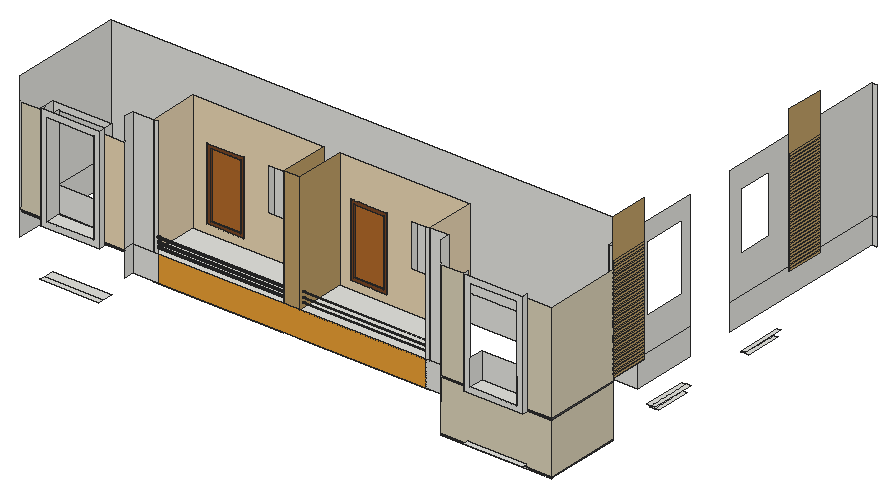
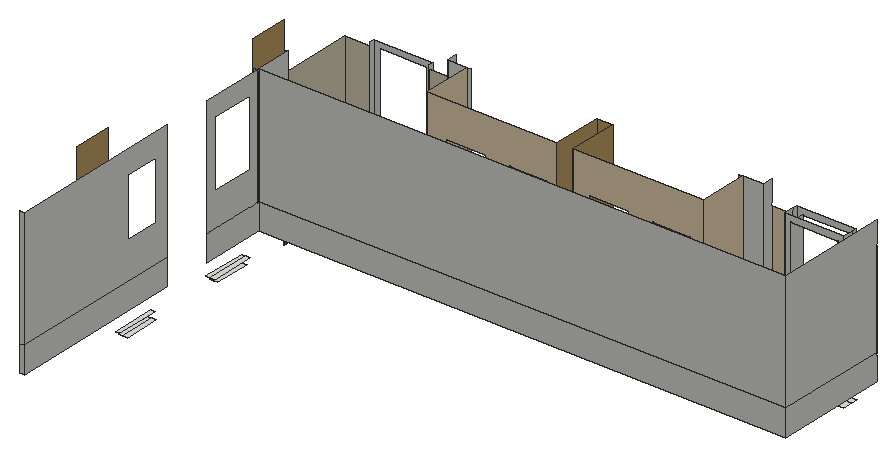
# SketchUp Ruby script. Lengths in inches.
U = 1.inch
M = Sketchup.active_model
def pt(a) = Geom::Point3d.new(a.map { |v| v * U })
def face(e, loops, mat)
  f = e.add_face(loops[0].map { |a| pt(a) })
  loops[1..].each { |l| e.add_face(l.map { |a| pt(a) }).erase! }
  f.material = f.back_material = mat if mat
  f
end
# faces: each face lists its corners as indices into pts; further lists are holes
def faces(e, pts, list, mat = nil) = list.each { |f| face(e, (f[0].is_a?(Array) ? f : [f]).map { |l| l.map { |i| pts[i] } }, mat) }
# xy, xz, yz: faces in a plane at the given z, y or x. An outline is a flat list of corners, or four numbers for a rectangle; further outlines are holes
def ring(l) = l.size == 4 ? [[l[0], l[1]], [l[2], l[1]], [l[2], l[3]], [l[0], l[3]]] : l.each_slice(2).to_a
def flat(e, list, mat, &to3) = list.each { |f| face(e, (f[0].is_a?(Array) ? f : [f]).map { |l| ring(l).map { |u, v| to3.(u, v) } }, mat) }
def xy(e, z, list, mat = nil) = flat(e, list, mat) { |x, y| [x, y, z] }
def xz(e, y, list, mat = nil) = flat(e, list, mat) { |x, z| [x, y, z] }
def yz(e, x, list, mat = nil) = flat(e, list, mat) { |y, z| [x, y, z] }
def lines(e, pts, list) = list.each { |a, b| e.add_line(pt(pts[a]), pt(pts[b])) }
# prism: a flat outline (further loops are holes) pulled along v
def prism(e, loops, v, mat = nil)
  f = face(e, loops, mat); d = Geom::Vector3d.new(v.map { |x| x * U })
  f.pushpull(f.normal.samedirection?(d) ? d.length : -d.length)
end
def box(e, o, s, mat = nil) = prism(e, [[o, [o[0] + s[0], o[1], o[2]], [o[0] + s[0], o[1] + s[1], o[2]], [o[0], o[1] + s[1], o[2]]]], [0, 0, s[2]], mat)
def at(x, y, z, deg = 0) = Geom::Transformation.translation(pt([x, y, z])) * Geom::Transformation.rotation(ORIGIN, Z_AXIS, deg.degrees)
def axes(o, x, y, z) = Geom::Transformation.new([*x, 0, *y, 0, *z, 0, *pt(o).to_a, 1])
def part(name) = M.definitions.add(name)
# library, detail: a bought-in or finely detailed component or shape, given as its bounding box
def library(name, o, s) = part(name).tap { |d| box(d.entities, o, s) }
def detail(e, o, s) = box(e.add_group.entities, o, s)
def put(e, d, t, mat = nil) = e.add_instance(d, t).tap { |i| i.material = mat if mat }
def group(e, t, mat = nil) = e.add_group.tap { |g| g.transformation = t; g.material = mat if mat }.entities
root = M.entities
M.materials.add("Generic").color = [191, 159, 103]
M.materials.add("Generic\#1").color = [233, 159, 52]
M.materials.add("Generic\#2").color = [235, 215, 180]
M.materials.add("Generic\#3").color = [218, 209, 183]
M.materials.add("[Color M06]").color = [86, 86, 86]
M.materials.add("[Wood Bamboo]").color = [177, 105, 43]
M.materials.add("[Wood Veneer 01]").color = [120, 70, 37]
c1 = part("Group\#5")
xy(c1.entities,0,[[0,0,1,57.75]])
xy(c1.entities,2.57,[[0,0,1,57.75]])
xz(c1.entities,0,[[0,0,1,2.57]])
xz(c1.entities,57.75,[[0,0,1,2.57]])
yz(c1.entities,1,[[0,0,57.75,2.57]])
c2 = part("Group\#6")
put(c2.entities,c1,at(0,0,4.75))
put(c2.entities,c1,at(0,0,0))
put(c2.entities,c1,at(0,0,19))
put(c2.entities,c1,at(0,0,28.5))
put(c2.entities,c1,at(0,0,133))
put(c2.entities,c1,at(0,0,152))
put(c2.entities,c1,at(0,0,128.25))
put(c2.entities,c1,at(0,0,9.5))
put(c2.entities,c1,at(0,0,123.5))
put(c2.entities,c1,at(0,0,114))
put(c2.entities,c1,at(0,0,147.25))
put(c2.entities,c1,at(0,0,118.75))
put(c2.entities,c1,at(0,0,142.5))
put(c2.entities,c1,at(0,0,109.25))
put(c2.entities,c1,at(0,0,137.75))
put(c2.entities,c1,at(0,0,104.5))
put(c2.entities,c1,at(0,0,99.75))
put(c2.entities,c1,at(0,0,95))
put(c2.entities,c1,at(0,0,85.5))
put(c2.entities,c1,at(0,0,80.75))
put(c2.entities,c1,at(0,0,90.25))
put(c2.entities,c1,at(0,0,76))
put(c2.entities,c1,at(0,0,71.25))
put(c2.entities,c1,at(0,0,38))
put(c2.entities,c1,at(0,0,14.25))
put(c2.entities,c1,at(0,0,33.25))
put(c2.entities,c1,at(0,0,57))
put(c2.entities,c1,at(0,0,23.75))
put(c2.entities,c1,at(0,0,61.75))
put(c2.entities,c1,at(0,0,156.75))
put(c2.entities,c1,at(0,0,47.5))
put(c2.entities,c1,at(0,0,52.25))
put(c2.entities,c1,at(0,0,42.75))
put(c2.entities,c1,at(0,0,66.5))
c3 = part("Group\#4")
xy(c3.entities,0,[[0,0,55.6875,6]],"[Wood Veneer 01]")
xy(c3.entities,4.75,[[4.75,0,50.9375,3]],"[Wood Veneer 01]")
xy(c3.entities,105.5,[[4.75,0,50.9375,3]],"[Wood Veneer 01]")
xy(c3.entities,110.25,[[0,0,55.6875,6]],"[Wood Veneer 01]")
xz(c3.entities,0,[[[0,0,55.6875,110.25],[4.75,4.75,50.9375,105.5]]],"[Wood Veneer 01]")
xz(c3.entities,3,[[4.75,4.75,50.9375,105.5]],"[Wood Bamboo]")
xz(c3.entities,6,[[0,0,55.6875,110.25]],"[Wood Bamboo]")
yz(c3.entities,0,[[0,0,6,110.25]],"[Wood Veneer 01]")
yz(c3.entities,4.75,[[0,4.75,3,105.5]],"[Wood Veneer 01]")
yz(c3.entities,50.9375,[[0,4.75,3,105.5]],"[Wood Veneer 01]")
yz(c3.entities,55.6875,[[0,0,6,110.25]],"[Wood Veneer 01]")
xy(root,574.59,[[641.55,68.5,682.51,69.9375],[771.75,68.5,802.875,69.9375],[802.875,68.5,809.375,69.9375],[807.9375,69.9375,809.375,185.01]])
xy(root,574.63,[[307.73,150.125,367.625,158.75],[523.54,150.125,583.4375,158.75]])
xy(root,577.59,[[641.55,68.5,682.51,69.9375],[771.75,68.5,809.375,69.9375],[807.9375,69.9375,809.375,185.01]])
xy(root,578.68,[[40.68,60.5625,129.91,68.5],[40.68,68.5,129.91,83.8125]])
xy(root,581.34,[[682.51,60.5625,771.75,68.5]])
xy(root,584.25,[[802.875,263.64,809.375,317.96],[809.375,263.64,815.3125,317.96],[802.875,434.88,809.375,489.19],[809.375,434.88,815.3125,489.19]])
xy(root,590.66,[[802.875,257.24,809.375,324.36],[809.375,257.24,815.3125,324.36],[809.375,428.47,815.3125,495.59]])
xy(root,619.5,[[193.83,83.8125,391.53,158.75],[415.53,83.8125,613.23,158.75]])
xy(root,651.7,[[41.1,60.5625,130.34,68.5],[41.1,68.5,130.34,83.8125]])
xy(root,652.32,[[682.51,60.5625,771.75,68.5]])
xy(root,653.5625,[[641.55,68.5,682.51,69.9375],[771.75,68.5,802.875,69.9375],[802.875,68.5,807.9375,69.9375],[807.9375,68.5,809.375,185.01]])
xy(root,655.14,[[4.1875,68.5,41.1,69.9375],[130.34,68.5,162.33,69.9375]])
xy(root,656.5625,[[641.55,68.5,682.51,69.9375],[771.75,68.5,807.9375,69.9375],[807.9375,68.5,809.375,185.01]])
xy(root,658.14,[[4.1875,68.5,41.1,69.9375],[130.34,68.5,162.33,69.9375]])
xy(root,659.25,[[193.83,83.8125,391.53,158.75],[415.53,83.8125,613.23,158.75],[802.875,185.01,809.375,242.76]])
xy(root,660.6,[[50,60.5625,121.4375,83.8125]])
xy(root,661.22,[[691.41,60.5625,762.85,83.8125]])
xy(root,672.0625,[[215.38,158.75,271.07,214.75],[432.26,158.75,487.94,214.75]])
xz(root,60.5625,[[[41.1,651.7,130.34,811.1],[50,660.6,121.4375,802.2]],[[682.51,652.32,771.75,811.71],[691.41,661.22,762.85,802.81]]])
xz(root,68.5,[[682.51,574.59,771.75,577.59],[682.51,653.5625,771.75,656.5625],[129.35,655.14,130.34,658.14]])
xz(root,68.5,[[130.34,658.14,162.33,803.75]],"Generic\#2")
xz(root,68.5,[[641.55,577.59,682.51,577.59,682.51,581.34,771.75,581.34,771.75,577.59,809.375,577.59,809.375,653.5625,771.75,653.5625,771.75,652.32,682.51,652.32,682.51,653.5625,641.55,653.5625],[641.55,656.5625,682.51,806.5],[771.75,656.5625,809.375,806.5],[4.1875,658.14,41.1,803.75]],"Generic\#3")
xz(root,69.9375,[[641.55,574.59,682.51,577.59],[771.75,574.59,807.9375,577.59],[641.55,653.5625,682.51,656.5625],[771.75,653.5625,807.9375,656.5625],[4.1875,655.14,41.1,658.14],
  [130.34,655.14,162.33,658.14]],"[Color M06]")
xz(root,83.8125,[[162.33,619.5,200.02,659.25],[607.05,619.5,641.55,659.25],[[41.1,651.7,130.34,811.1],[50,660.6,121.4375,802.2]],[162.33,659.25,193.83,839.25],[193.83,659.25,200.02,839.25],
  [607.05,659.25,613.23,839.25],[613.23,659.25,641.55,839.25],[50,660.6,121.4375,699.45],[691.41,661.22,762.85,700.06]])
xz(root,83.8125,[[391.53,659.25,415.53,839.25]],"Generic")
xz(root,83.8125,[[200.02,619.5,607.05,659.25]],"Generic\#1")
xz(root,158.75,[[[193.83,659.25,391.53,839.25],[215.38,672.0625,271.07,782.3125],[307.73,719.55,367.625,785.38]],[[415.53,659.25,613.23,839.25],[432.26,672.0625,487.94,782.3125],[524.6,719.55,584.5,785.38]]],"Generic\#2")
xz(root,185.01,[[807.9375,574.59,809.375,577.59],[807.9375,653.5625,809.375,656.5625],[802.875,659.25,809.375,659.25,809.375,806.5,807.9375,806.5,807.9375,809.5,809.375,809.5,809.375,839.25,802.875,839.25]])
xz(root,214.75,[[215.38,672.0625,271.07,782.3125],[432.26,672.0625,487.94,782.3125]])
xz(root,239.73,[[4.1875,619.5,802.875,659.25],[4.1875,659.25,802.875,839.25]])
xz(root,242.76,[[802.875,659.25,809.375,839.25]])
xz(root,683.8125,[[802.875,619.5,809.375,659.25],[802.875,659.25,809.375,839.25]])
yz(root,4.1875,[[68.5,619.5,68.5,655.14,69.9375,655.14,69.9375,658.14,68.5,658.14,68.5,659.25,239.73,659.25,239.73,619.5],[68.5,659.25,68.5,803.75,69.9375,803.75,69.9375,806.75,68.5,806.75,68.5,839.25,239.73,839.25,239.73,659.25]])
yz(root,41.1,[[60.5625,651.7,68.5,651.7,68.5,655.14,69.9375,655.14,69.9375,658.14,68.5,658.14,68.5,803.75,69.9375,803.75,69.9375,806.75,68.5,806.75,68.5,811.1,60.5625,811.1],[68.5,651.7,83.8125,651.7,83.8125,811.1,68.5,811.1,68.5,806.75,69.9375,806.75,69.9375,803.75,68.5,803.75,68.5,658.14,69.9375,658.14,69.9375,655.14,68.5,655.14]])
yz(root,50,[[60.5625,660.6,83.8125,802.2]])
yz(root,121.4375,[[60.5625,660.6,83.8125,802.2]])
yz(root,130.34,[[60.5625,651.7,68.5,811.1],[68.5,651.7,68.5,655.14,69.9375,655.14,69.9375,658.14,68.5,658.14,68.5,803.75,69.9375,803.75,69.9375,806.75,68.5,806.75,68.5,811.1,83.8125,811.1,83.8125,651.7],[68.5,655.14,69.9375,658.14]])
yz(root,162.33,[[68.5,619.5,68.5,655.14,69.9375,655.14,69.9375,658.14,68.5,658.14,68.5,659.25,83.8125,659.25,83.8125,619.5],[68.5,659.25,68.5,803.75,69.9375,803.75,69.9375,806.75,68.5,806.75,68.5,839.25,83.8125,839.25,83.8125,659.25]])
yz(root,193.83,[[[83.8125,659.25,158.75,839.25],[90.04,690.15,89.73,690.1875,89.44,690.31,89.2,690.49,89.01,690.74,88.89,691.03,88.85,691.33,88.89,691.64,89.01,691.93,89.2,692.17,89.44,692.36,89.73,692.48,90.04,692.52,90.35,692.48,90.63,692.36,90.88,692.17,91.07,691.93,91.18,691.64,91.23,691.33,91.18,691.03,91.07,690.74,90.88,690.49,90.63,690.31,90.35,690.1875],[90.04,683.58,89.73,683.625,89.44,683.74,89.2,683.93,89.01,684.18,88.89,684.46,88.85,684.77,88.89,685.08,89.01,685.36,89.2,685.61,89.44,685.8,89.73,685.92,90.04,685.96,90.35,685.92,90.63,685.8,90.88,685.61,91.07,685.36,91.18,685.08,91.23,684.77,91.18,684.46,91.07,684.18,90.88,683.93,90.63,683.74,90.35,683.625],[90.04,676.58,89.73,676.625,89.44,676.74,89.2,676.93,89.01,677.18,88.89,677.46,88.85,677.77,88.89,678.08,89.01,678.36,89.2,678.61,89.44,678.8,89.73,678.92,90.04,678.96,90.35,678.92,90.63,678.8,90.88,678.61,91.07,678.36,91.18,678.08,91.23,677.77,91.18,677.46,91.07,677.18,90.88,676.93,90.63,676.74,90.35,676.625],[90.04,669.58,89.73,669.625,89.44,669.74,89.2,669.93,89.01,670.18,88.89,670.46,88.85,670.77,88.89,671.08,89.01,671.36,89.2,671.61,89.44,671.8,89.73,671.92,90.04,671.96,90.35,671.92,90.63,671.8,90.88,671.61,91.07,671.36,91.18,671.08,91.23,670.77,91.18,670.46,91.07,670.18,90.88,669.93,90.63,669.74,90.35,669.625],[90.04,662.9,89.73,662.9375,89.44,663.06,89.2,663.24,89.01,663.49,88.89,663.78,88.85,664.08,88.89,664.39,89.01,664.68,89.2,664.92,89.44,665.11,89.73,665.23,90.04,665.27,90.35,665.23,90.63,665.11,90.88,664.92,91.07,664.68,91.18,664.39,91.23,664.08,91.18,663.78,91.07,663.49,90.88,663.24,90.63,663.06,90.35,662.9375]]],"Generic\#2")
yz(root,215.38,[[158.75,672.0625,214.75,782.3125]])
yz(root,271.07,[[158.75,672.0625,214.75,782.3125]])
yz(root,391.53,[[[83.8125,659.25,158.75,839.25],[90.04,690.15,90.35,690.1875,90.63,690.31,90.88,690.49,91.07,690.74,91.18,691.03,91.23,691.33,91.18,691.64,91.07,691.93,90.88,692.17,90.63,692.36,90.35,692.48,90.04,692.52,89.73,692.48,89.44,692.36,89.2,692.17,89.01,691.93,88.89,691.64,88.85,691.33,88.89,691.03,89.01,690.74,89.2,690.49,89.44,690.31,89.73,690.1875],[90.04,683.58,90.35,683.625,90.63,683.74,90.88,683.93,91.07,684.18,91.18,684.46,91.23,684.77,91.18,685.08,91.07,685.36,90.88,685.61,90.63,685.8,90.35,685.92,90.04,685.96,89.73,685.92,89.44,685.8,89.2,685.61,89.01,685.36,88.89,685.08,88.85,684.77,88.89,684.46,89.01,684.18,89.2,683.93,89.44,683.74,89.73,683.625],[90.04,676.58,90.35,676.625,90.63,676.74,90.88,676.93,91.07,677.18,91.18,677.46,91.23,677.77,91.18,678.08,91.07,678.36,90.88,678.61,90.63,678.8,90.35,678.92,90.04,678.96,89.73,678.92,89.44,678.8,89.2,678.61,89.01,678.36,88.89,678.08,88.85,677.77,88.89,677.46,89.01,677.18,89.2,676.93,89.44,676.74,89.73,676.625],[90.04,669.58,90.35,669.625,90.63,669.74,90.88,669.93,91.07,670.18,91.18,670.46,91.23,670.77,91.18,671.08,91.07,671.36,90.88,671.61,90.63,671.8,90.35,671.92,90.04,671.96,89.73,671.92,89.44,671.8,89.2,671.61,89.01,671.36,88.89,671.08,88.85,670.77,88.89,670.46,89.01,670.18,89.2,669.93,89.44,669.74,89.73,669.625],[90.04,662.9,90.35,662.9375,90.63,663.06,90.88,663.24,91.07,663.49,91.18,663.78,91.23,664.08,91.18,664.39,91.07,664.68,90.88,664.92,90.63,665.11,90.35,665.23,90.04,665.27,89.73,665.23,89.44,665.11,89.2,664.92,89.01,664.68,88.89,664.39,88.85,664.08,88.89,663.78,89.01,663.49,89.2,663.24,89.44,663.06,89.73,662.9375]]],"Generic")
yz(root,415.53,[[[83.8125,659.25,158.75,839.25],[89.21,680.46,89.0625,680.48,88.93,680.54,88.8125,680.625,88.72,680.74,88.67,680.88,88.65,681.02,88.67,681.17,88.72,681.31,88.8125,681.42,88.93,681.51,89.0625,681.57,89.21,681.59,89.36,681.57,89.49,681.51,89.61,681.42,89.7,681.31,89.75,681.17,89.77,681.02,89.75,680.88,89.7,680.74,89.61,680.625,89.49,680.54,89.36,680.48],[89.21,672.96,89.0625,672.98,88.93,673.04,88.8125,673.125,88.72,673.24,88.67,673.38,88.65,673.52,88.67,673.67,88.72,673.81,88.8125,673.92,88.93,674.01,89.0625,674.07,89.21,674.09,89.36,674.07,89.49,674.01,89.61,673.92,89.7,673.81,89.75,673.67,89.77,673.52,89.75,673.38,89.7,673.24,89.61,673.125,89.49,673.04,89.36,672.98],[89.21,665.59,89.0625,665.61,88.93,665.66,88.8125,665.75,88.72,665.87,88.67,666,88.65,666.15,88.67,666.29,88.72,666.43,88.8125,666.55,88.93,666.64,89.0625,666.69,89.21,666.71,89.36,666.69,89.49,666.64,89.61,666.55,89.7,666.43,89.75,666.29,89.77,666.15,89.75,666,89.7,665.87,89.61,665.75,89.49,665.66,89.36,665.61],[89.21,695.4,89.0625,695.42,88.93,695.47,88.8125,695.5625,88.72,695.68,88.67,695.82,88.65,695.96,88.67,696.11,88.72,696.24,88.8125,696.36,88.93,696.45,89.0625,696.51,89.21,696.52,89.36,696.51,89.49,696.45,89.61,696.36,89.7,696.24,89.75,696.11,89.77,695.96,89.75,695.82,89.7,695.68,89.61,695.5625,89.49,695.47,89.36,695.42],[89.21,687.96,89.0625,687.98,88.93,688.04,88.8125,688.125,88.72,688.24,88.67,688.38,88.65,688.52,88.67,688.67,88.72,688.81,88.8125,688.92,88.93,689.01,89.0625,689.07,89.21,689.09,89.36,689.07,89.49,689.01,89.61,688.92,89.7,688.81,89.75,688.67,89.77,688.52,89.75,688.38,89.7,688.24,89.61,688.125,89.49,688.04,89.36,687.98]]],"Generic")
yz(root,432.26,[[158.75,672.0625,214.75,782.3125]])
yz(root,487.94,[[158.75,672.0625,214.75,782.3125]])
yz(root,613.23,[[[83.8125,659.25,158.75,839.25],[89.21,680.46,89.36,680.48,89.49,680.54,89.61,680.625,89.7,680.74,89.75,680.88,89.77,681.02,89.75,681.17,89.7,681.31,89.61,681.42,89.49,681.51,89.36,681.57,89.21,681.59,89.0625,681.57,88.93,681.51,88.8125,681.42,88.72,681.31,88.67,681.17,88.65,681.02,88.67,680.88,88.72,680.74,88.8125,680.625,88.93,680.54,89.0625,680.48],[89.21,672.96,89.36,672.98,89.49,673.04,89.61,673.125,89.7,673.24,89.75,673.38,89.77,673.52,89.75,673.67,89.7,673.81,89.61,673.92,89.49,674.01,89.36,674.07,89.21,674.09,89.0625,674.07,88.93,674.01,88.8125,673.92,88.72,673.81,88.67,673.67,88.65,673.52,88.67,673.38,88.72,673.24,88.8125,673.125,88.93,673.04,89.0625,672.98],[89.21,665.59,89.36,665.61,89.49,665.66,89.61,665.75,89.7,665.87,89.75,666,89.77,666.15,89.75,666.29,89.7,666.43,89.61,666.55,89.49,666.64,89.36,666.69,89.21,666.71,89.0625,666.69,88.93,666.64,88.8125,666.55,88.72,666.43,88.67,666.29,88.65,666.15,88.67,666,88.72,665.87,88.8125,665.75,88.93,665.66,89.0625,665.61],[89.21,695.4,89.36,695.42,89.49,695.47,89.61,695.5625,89.7,695.68,89.75,695.82,89.77,695.96,89.75,696.11,89.7,696.24,89.61,696.36,89.49,696.45,89.36,696.51,89.21,696.52,89.0625,696.51,88.93,696.45,88.8125,696.36,88.72,696.24,88.67,696.11,88.65,695.96,88.67,695.82,88.72,695.68,88.8125,695.5625,88.93,695.47,89.0625,695.42],[89.21,687.96,89.36,687.98,89.49,688.04,89.61,688.125,89.7,688.24,89.75,688.38,89.77,688.52,89.75,688.67,89.7,688.81,89.61,688.92,89.49,689.01,89.36,689.07,89.21,689.09,89.0625,689.07,88.93,689.01,88.8125,688.92,88.72,688.81,88.67,688.67,88.65,688.52,88.67,688.38,88.72,688.24,88.8125,688.125,88.93,688.04,89.0625,687.98]]],"Generic\#2")
yz(root,641.55,[[68.5,619.5,83.8125,619.5,83.8125,659.25,68.5,659.25,68.5,656.5625,69.9375,656.5625,69.9375,653.5625,68.5,653.5625],[68.5,659.25,83.8125,659.25,83.8125,839.25,68.5,839.25,68.5,809.5,69.9375,809.5,69.9375,806.5,68.5,806.5]])
yz(root,682.51,[[68.5,574.59,69.9375,577.59],[60.5625,652.32,68.5,811.71],[68.5,653.5625,69.9375,656.5625]])
yz(root,691.41,[[60.5625,661.22,83.8125,700.06]])
yz(root,762.85,[[60.5625,661.22,83.8125,700.06]])
yz(root,771.75,[[68.5,574.59,69.9375,577.59],[60.5625,652.32,68.5,811.71],[68.5,653.5625,69.9375,656.5625]])
yz(root,802.875,[[239.73,619.5,338.625,659.25],[413.6875,619.5,683.8125,659.25],[185.01,659.25,239.73,839.25],[239.73,659.25,242.76,839.25],[[242.76,659.25,338.625,839.25],[257.24,710.22,324.36,810.91]],
  [[413.6875,659.25,683.8125,839.25],[434.88,716.625,489.19,804.5]]])
yz(root,807.9375,[[69.9375,574.59,185.01,577.59],[69.9375,653.5625,185.01,656.5625]],"[Color M06]")
yz(root,809.375,[[185.01,659.25,242.76,879],[518.09,659.25,575.84,879]],"Generic")
yz(root,809.375,[[68.5,577.59,185.01,653.5625],[68.5,656.5625,185.01,806.5]],"Generic\#3")
p = [[193.83,89.44,663.06],[193.83,89.73,662.9375],[391.53,89.73,662.9375],[391.53,89.44,663.06],[193.83,90.04,662.9],[391.53,90.04,662.9],
  [193.83,90.35,662.9375],[391.53,90.35,662.9375],[193.83,90.63,663.06],[391.53,90.63,663.06],[193.83,89.2,663.24],[391.53,89.2,663.24],
  [193.83,90.88,663.24],[391.53,90.88,663.24],[193.83,89.01,663.49],[391.53,89.01,663.49],[193.83,91.07,663.49],[391.53,91.07,663.49],
  [193.83,88.89,663.78],[391.53,88.89,663.78],[193.83,91.18,663.78],[391.53,91.18,663.78],[193.83,88.85,664.08],[391.53,88.85,664.08],
  [193.83,91.23,664.08],[391.53,91.23,664.08],[193.83,88.89,664.39],[391.53,88.89,664.39],[193.83,91.18,664.39],[391.53,91.18,664.39],
  [193.83,89.01,664.68],[391.53,89.01,664.68],[193.83,91.07,664.68],[391.53,91.07,664.68],[193.83,89.2,664.92],[391.53,89.2,664.92],
  [193.83,90.88,664.92],[391.53,90.88,664.92],[193.83,89.44,665.11],[391.53,89.44,665.11],[193.83,90.63,665.11],[391.53,90.63,665.11],
  [193.83,89.73,665.23],[391.53,89.73,665.23],[193.83,90.35,665.23],[391.53,90.35,665.23],[193.83,90.04,665.27],[391.53,90.04,665.27],
  [415.53,88.93,665.66],[415.53,89.0625,665.61],[613.23,89.0625,665.61],[613.23,88.93,665.66],[415.53,89.21,665.59],[613.23,89.21,665.59],
  [415.53,89.36,665.61],[613.23,89.36,665.61],[415.53,89.49,665.66],[613.23,89.49,665.66],[415.53,88.8125,665.75],[613.23,88.8125,665.75],
  [415.53,89.61,665.75],[613.23,89.61,665.75],[415.53,88.72,665.87],[613.23,88.72,665.87],[415.53,89.7,665.87],[613.23,89.7,665.87],
  [415.53,88.67,666],[613.23,88.67,666],[415.53,89.75,666],[613.23,89.75,666],[415.53,88.65,666.15],[613.23,88.65,666.15],
  [415.53,89.77,666.15],[613.23,89.77,666.15],[415.53,88.67,666.29],[613.23,88.67,666.29],[415.53,89.75,666.29],[613.23,89.75,666.29],
  [415.53,88.72,666.43],[613.23,88.72,666.43],[415.53,89.7,666.43],[613.23,89.7,666.43],[415.53,88.8125,666.55],[613.23,88.8125,666.55],
  [415.53,89.61,666.55],[613.23,89.61,666.55],[415.53,88.93,666.64],[613.23,88.93,666.64],[415.53,89.49,666.64],[613.23,89.49,666.64],
  [415.53,89.0625,666.69],[613.23,89.0625,666.69],[415.53,89.36,666.69],[613.23,89.36,666.69],[415.53,89.21,666.71],[613.23,89.21,666.71],
  [193.83,89.44,669.74],[193.83,89.73,669.625],[391.53,89.73,669.625],[391.53,89.44,669.74],[193.83,90.04,669.58],[391.53,90.04,669.58],
  [193.83,90.35,669.625],[391.53,90.35,669.625],[193.83,90.63,669.74],[391.53,90.63,669.74],[193.83,89.2,669.93],[391.53,89.2,669.93],
  [193.83,90.88,669.93],[391.53,90.88,669.93],[193.83,89.01,670.18],[391.53,89.01,670.18],[193.83,91.07,670.18],[391.53,91.07,670.18],
  [193.83,88.89,670.46],[391.53,88.89,670.46],[193.83,91.18,670.46],[391.53,91.18,670.46],[193.83,88.85,670.77],[391.53,88.85,670.77],
  [193.83,91.23,670.77],[391.53,91.23,670.77],[193.83,88.89,671.08],[391.53,88.89,671.08],[193.83,91.18,671.08],[391.53,91.18,671.08],
  [193.83,89.01,671.36],[391.53,89.01,671.36],[193.83,91.07,671.36],[391.53,91.07,671.36],[193.83,89.2,671.61],[391.53,89.2,671.61],
  [193.83,90.88,671.61],[391.53,90.88,671.61],[193.83,89.44,671.8],[391.53,89.44,671.8],[193.83,90.63,671.8],[391.53,90.63,671.8],
  [193.83,89.73,671.92],[391.53,89.73,671.92],[193.83,90.35,671.92],[391.53,90.35,671.92],[193.83,90.04,671.96],[391.53,90.04,671.96],
  [415.53,88.8125,673.125],[415.53,88.93,673.04],[613.23,88.93,673.04],[613.23,88.8125,673.125],[415.53,89.0625,672.98],[613.23,89.0625,672.98],
  [415.53,89.21,672.96],[613.23,89.21,672.96],[415.53,89.36,672.98],[613.23,89.36,672.98],[415.53,89.49,673.04],[613.23,89.49,673.04],
  [415.53,89.61,673.125],[613.23,89.61,673.125],[415.53,88.72,673.24],[613.23,88.72,673.24],[415.53,89.7,673.24],[613.23,89.7,673.24],
  [415.53,88.67,673.38],[613.23,88.67,673.38],[415.53,89.75,673.38],[613.23,89.75,673.38],[415.53,88.65,673.52],[613.23,88.65,673.52],
  [415.53,89.77,673.52],[613.23,89.77,673.52],[415.53,88.67,673.67],[613.23,88.67,673.67],[415.53,89.75,673.67],[613.23,89.75,673.67],
  [415.53,88.72,673.81],[613.23,88.72,673.81],[415.53,89.7,673.81],[613.23,89.7,673.81],[415.53,88.8125,673.92],[613.23,88.8125,673.92],
  [415.53,89.61,673.92],[613.23,89.61,673.92],[415.53,88.93,674.01],[613.23,88.93,674.01],[415.53,89.49,674.01],[613.23,89.49,674.01],
  [415.53,89.0625,674.07],[613.23,89.0625,674.07],[415.53,89.36,674.07],[613.23,89.36,674.07],[415.53,89.21,674.09],[613.23,89.21,674.09],
  [193.83,89.44,676.74],[193.83,89.73,676.625],[391.53,89.73,676.625],[391.53,89.44,676.74],[193.83,90.04,676.58],[391.53,90.04,676.58],
  [193.83,90.35,676.625],[391.53,90.35,676.625],[193.83,90.63,676.74],[391.53,90.63,676.74],[193.83,89.2,676.93],[391.53,89.2,676.93],
  [193.83,90.88,676.93],[391.53,90.88,676.93],[193.83,89.01,677.18],[391.53,89.01,677.18],[193.83,91.07,677.18],[391.53,91.07,677.18],
  [193.83,88.89,677.46],[391.53,88.89,677.46],[193.83,91.18,677.46],[391.53,91.18,677.46],[193.83,88.85,677.77],[391.53,88.85,677.77],
  [193.83,91.23,677.77],[391.53,91.23,677.77],[193.83,88.89,678.08],[391.53,88.89,678.08],[193.83,91.18,678.08],[391.53,91.18,678.08],
  [193.83,89.01,678.36],[391.53,89.01,678.36],[193.83,91.07,678.36],[391.53,91.07,678.36],[193.83,89.2,678.61],[391.53,89.2,678.61],
  [193.83,90.88,678.61],[391.53,90.88,678.61],[193.83,89.44,678.8],[391.53,89.44,678.8],[193.83,90.63,678.8],[391.53,90.63,678.8],
  [193.83,89.73,678.92],[391.53,89.73,678.92],[193.83,90.35,678.92],[391.53,90.35,678.92],[193.83,90.04,678.96],[391.53,90.04,678.96],
  [415.53,88.8125,680.625],[415.53,88.93,680.54],[613.23,88.93,680.54],[613.23,88.8125,680.625],[415.53,89.0625,680.48],[613.23,89.0625,680.48],
  [415.53,89.21,680.46],[613.23,89.21,680.46],[415.53,89.36,680.48],[613.23,89.36,680.48],[415.53,89.49,680.54],[613.23,89.49,680.54],
  [415.53,89.61,680.625],[613.23,89.61,680.625],[415.53,88.72,680.74],[613.23,88.72,680.74],[415.53,89.7,680.74],[613.23,89.7,680.74],
  [415.53,88.67,680.88],[613.23,88.67,680.88],[415.53,89.75,680.88],[613.23,89.75,680.88],[415.53,88.65,681.02],[613.23,88.65,681.02],
  [415.53,89.77,681.02],[613.23,89.77,681.02],[415.53,88.67,681.17],[613.23,88.67,681.17],[415.53,89.75,681.17],[613.23,89.75,681.17],
  [415.53,88.72,681.31],[613.23,88.72,681.31],[415.53,89.7,681.31],[613.23,89.7,681.31],[415.53,88.8125,681.42],[613.23,88.8125,681.42],
  [415.53,89.61,681.42],[613.23,89.61,681.42],[415.53,88.93,681.51],[613.23,88.93,681.51],[415.53,89.49,681.51],[613.23,89.49,681.51],
  [415.53,89.0625,681.57],[613.23,89.0625,681.57],[415.53,89.36,681.57],[613.23,89.36,681.57],[415.53,89.21,681.59],[613.23,89.21,681.59],
  [802.875,68.5,619.5],[802.875,185.01,619.5],[802.875,68.5,659.25],[802.875,185.01,659.25],[415.53,89.21,666.15],[613.23,89.21,666.15],
  [415.53,89.21,681.02],[613.23,89.21,681.02],[193.83,90.04,664.08],[391.53,90.04,664.08],[193.83,90.04,677.58],[391.53,90.04,677.58],
  [193.83,90.04,670.83],[391.53,90.04,670.83],[415.53,89.21,673.59],[613.23,89.21,673.59]]
faces(root,p,[[0,1,2,3],[1,4,5,2],[4,6,7,5],[6,8,9,7],[10,0,3,11],[8,12,13,9],[14,10,11,15],[12,16,17,13],
  [18,14,15,19],[16,20,21,17],[22,18,19,23],[20,24,25,21],[26,22,23,27],[24,28,29,25],[30,26,27,31],[28,32,33,29],
  [34,30,31,35],[32,36,37,33],[38,34,35,39],[36,40,41,37],[42,38,39,43],[40,44,45,41],[46,42,43,47],[44,46,47,45],
  [48,49,50,51],[49,52,53,50],[52,54,55,53],[54,56,57,55],[58,48,51,59],[56,60,61,57],[62,58,59,63],[60,64,65,61],
  [66,62,63,67],[64,68,69,65],[70,66,67,71],[68,72,73,69],[74,70,71,75],[72,76,77,73],[78,74,75,79],[76,80,81,77],
  [82,78,79,83],[80,84,85,81],[86,82,83,87],[84,88,89,85],[90,86,87,91],[88,92,93,89],[94,90,91,95],[92,94,95,93],
  [96,97,98,99],[97,100,101,98],[100,102,103,101],[102,104,105,103],[106,96,99,107],[104,108,109,105],[110,106,107,111],[108,112,113,109],
  [114,110,111,115],[112,116,117,113],[118,114,115,119],[116,120,121,117],[122,118,119,123],[120,124,125,121],[126,122,123,127],[124,128,129,125],
  [130,126,127,131],[128,132,133,129],[134,130,131,135],[132,136,137,133],[138,134,135,139],[136,140,141,137],[142,138,139,143],[140,142,143,141],
  [144,145,146,147],[145,148,149,146],[148,150,151,149],[150,152,153,151],[152,154,155,153],[154,156,157,155],[158,144,147,159],[156,160,161,157],
  [162,158,159,163],[160,164,165,161],[166,162,163,167],[164,168,169,165],[170,166,167,171],[168,172,173,169],[174,170,171,175],[172,176,177,173],
  [178,174,175,179],[176,180,181,177],[182,178,179,183],[180,184,185,181],[186,182,183,187],[184,188,189,185],[190,186,187,191],[188,190,191,189],
  [192,193,194,195],[193,196,197,194],[196,198,199,197],[198,200,201,199],[202,192,195,203],[200,204,205,201],[206,202,203,207],[204,208,209,205],
  [210,206,207,211],[208,212,213,209],[214,210,211,215],[212,216,217,213],[218,214,215,219],[216,220,221,217],[222,218,219,223],[220,224,225,221],
  [226,222,223,227],[224,228,229,225],[230,226,227,231],[228,232,233,229],[234,230,231,235],[232,236,237,233],[238,234,235,239],[236,238,239,237],
  [240,241,242,243],[241,244,245,242],[244,246,247,245],[246,248,249,247],[248,250,251,249],[250,252,253,251],[254,240,243,255],[252,256,257,253],
  [258,254,255,259],[256,260,261,257],[262,258,259,263],[260,264,265,261],[266,262,263,267],[264,268,269,265],[270,266,267,271],[268,272,273,269],
  [274,270,271,275],[272,276,277,273],[278,274,275,279],[276,280,281,277],[282,278,279,283],[280,284,285,281],[286,282,283,287],[284,286,287,285]])
lines(root,p,[[288,289],[290,291],[292,293],[294,295],[296,297],[298,299],[300,301],[302,303]])
put(root,c2,at(809.4375,518.09,659.25),"Generic")
put(root,c2,at(809.375,185.01,660.7),"Generic")
put(root,c3,at(432.26,158.75,672.0625))
put(root,c3,at(215.38,158.75,672.0625))
